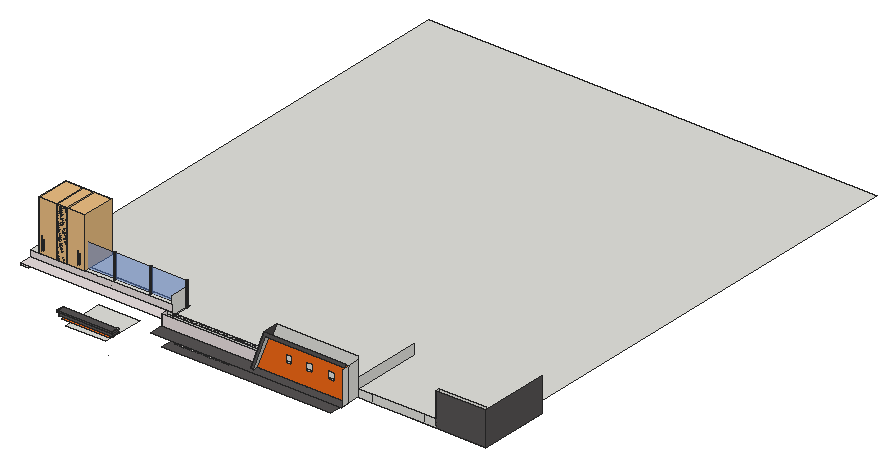
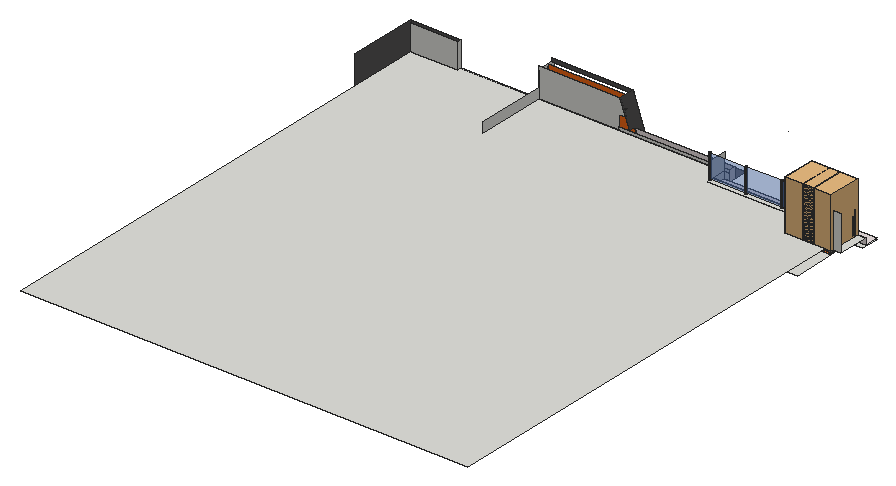
# SketchUp Ruby script. Lengths in inches.
U = 1.inch
M = Sketchup.active_model
def pt(a) = Geom::Point3d.new(a.map { |v| v * U })
def face(e, loops, mat)
  f = e.add_face(loops[0].map { |a| pt(a) })
  loops[1..].each { |l| e.add_face(l.map { |a| pt(a) }).erase! }
  f.material = f.back_material = mat if mat
  f
end
# faces: each face lists its corners as indices into pts; further lists are holes
def faces(e, pts, list, mat = nil) = list.each { |f| face(e, (f[0].is_a?(Array) ? f : [f]).map { |l| l.map { |i| pts[i] } }, mat) }
# xy, xz, yz: faces in a plane at the given z, y or x. An outline is a flat list of corners, or four numbers for a rectangle; further outlines are holes
def ring(l) = l.size == 4 ? [[l[0], l[1]], [l[2], l[1]], [l[2], l[3]], [l[0], l[3]]] : l.each_slice(2).to_a
def flat(e, list, mat, &to3) = list.each { |f| face(e, (f[0].is_a?(Array) ? f : [f]).map { |l| ring(l).map { |u, v| to3.(u, v) } }, mat) }
def xy(e, z, list, mat = nil) = flat(e, list, mat) { |x, y| [x, y, z] }
def xz(e, y, list, mat = nil) = flat(e, list, mat) { |x, z| [x, y, z] }
def yz(e, x, list, mat = nil) = flat(e, list, mat) { |y, z| [x, y, z] }
def lines(e, pts, list) = list.each { |a, b| e.add_line(pt(pts[a]), pt(pts[b])) }
# prism: a flat outline (further loops are holes) pulled along v
def prism(e, loops, v, mat = nil)
  f = face(e, loops, mat); d = Geom::Vector3d.new(v.map { |x| x * U })
  f.pushpull(f.normal.samedirection?(d) ? d.length : -d.length)
end
def box(e, o, s, mat = nil) = prism(e, [[o, [o[0] + s[0], o[1], o[2]], [o[0] + s[0], o[1] + s[1], o[2]], [o[0], o[1] + s[1], o[2]]]], [0, 0, s[2]], mat)
def at(x, y, z, deg = 0) = Geom::Transformation.translation(pt([x, y, z])) * Geom::Transformation.rotation(ORIGIN, Z_AXIS, deg.degrees)
def axes(o, x, y, z) = Geom::Transformation.new([*x, 0, *y, 0, *z, 0, *pt(o).to_a, 1])
def part(name) = M.definitions.add(name)
# library, detail: a bought-in or finely detailed component or shape, given as its bounding box
def library(name, o, s) = part(name).tap { |d| box(d.entities, o, s) }
def detail(e, o, s) = box(e.add_group.entities, o, s)
def put(e, d, t, mat = nil) = e.add_instance(d, t).tap { |i| i.material = mat if mat }
def group(e, t, mat = nil) = e.add_group.tap { |g| g.transformation = t; g.material = mat if mat }.entities
root = M.entities
M.materials.add("Generic").color = [243, 106, 23]
M.materials.add("Generic\#2").color = [87, 84, 84]
M.materials.add("Generic\#6").color = [174, 89, 41]
M.materials.add("Generic\#9").color = [233, 223, 223]
M.materials.add("[Translucent Glass Blue]").color = [100, 149, 237]
M.materials["[Translucent Glass Blue]"].alpha = 0.5
c1 = library("Plant",[-27.84,-31.84,-1.26],[68.28,70.82,154.38])
xy(root,207.139,[[115.793,121.25,154.87,162.1875]])
xy(root,211.524,[[112.407,121.25,158.881,127.4375]],"Generic")
xy(root,213.297,[[110.524,121.25,161.354,127.4375]],"Generic\#2")
xy(root,216.982,[[109.221,120,162.096,121.25]],"Generic\#2")
xy(root,217.98,[[109.165,120,162.04,127.4375]],"Generic\#2")
xy(root,231,[[220.539,107.5625,220.539,127.4375,381.97,127.4375,381.97,133.125,383.845,133.125,383.845,107.5625]],"Generic\#2")
xy(root,232.215,[[225.629,116.134,229.379,121.072],[231.317,116.134,235.067,121.072],[237.004,116.134,240.754,121.072],[242.692,116.134,246.442,121.072],[248.379,116.134,252.129,121.072],
  [254.067,116.134,257.817,121.072],[259.754,116.134,263.504,121.072],[265.442,116.134,269.192,121.072],[271.442,116.134,278.629,121.072]])
xy(root,237.6875,[[342.977,127.4375,342.977,133.364,220.539,133.364,220.539,168.255,342.977,168.255,342.977,194.75,385.914,194.75,385.914,133.125,381.97,133.125,381.97,127.4375]],"Generic\#6")
xy(root,240,[[302.78,111.75,306.093,115.8125],[302.78,115.8125,316.414,115.8125,316.414,127.4375,220.539,127.4375,220.539,120.9375,302.78,120.9375],[316.414,115.8125,394.852,127.4375],[209.664,120.9375,220.539,127.4375],[67.114,127.4375,75.375,143.9375],
  [220.539,127.4375,342.977,133.364],[381.97,127.4375,394.852,133.125],[394.852,127.4375,470.289,194.75],[[470.289,127.4375,518.6875,194.75],[472.756,133.845,475.694,136.783],[477.465,133.845,480.402,136.783],[482.59,133.845,485.527,136.783],[487.715,133.845,490.652,136.783],[492.84,133.845,495.777,136.783],[497.965,133.845,500.902,136.783],[503.09,133.845,506.027,136.783],[508.215,133.845,511.152,136.783]],[385.914,133.125,394.852,194.75]])
xy(root,240,[[209.664,107.5625,394.852,107.5625,394.852,115.8125,306.093,115.8125,306.093,111.75,302.78,111.75,302.78,120.9375,209.664,120.9375]],"Generic\#2")
xy(root,241.3125,[[80.9375,140.625,205.435,143.9375],[205.435,140.625,214.955,147.625]])
xy(root,241.3125,[[67.114,127.4375,214.955,140.625]],"Generic\#9")
xy(root,247.625,[[214.955,127.4375,470.289,127.4375,470.289,131.45,515.25,131.45,515.25,605.125,80.9375,605.125,80.9375,147.625,214.955,147.625,214.955,144.798,214.992,144.803,215.17,144.779,215.336,144.711,215.478,144.601,215.587,144.459,215.656,144.293,215.679,144.115,215.656,143.937,215.587,143.771,215.478,143.629,215.336,143.52,215.17,143.451,214.992,143.428,214.955,143.433],[67.114,140.625,214.955,140.625,214.955,143.433,214.814,143.451,214.648,143.52,214.506,143.629,214.396,143.771,214.328,143.937,214.304,144.115,214.328,144.293,214.396,144.459,180.656,144.291,180.679,144.115,180.656,143.937,180.587,143.771,180.478,143.629,180.336,143.52,180.17,143.451,179.992,143.428,179.814,143.451,179.648,143.52,179.506,143.629,179.396,143.771,179.328,143.937,179.304,144.115,179.327,144.285,145.866,144.118,145.867,144.115,145.843,143.937,145.775,143.771,145.665,143.629,145.523,143.52,145.357,143.451,145.179,143.428,145.001,143.451,144.836,143.52,144.693,143.629,144.584,143.771,144.515,143.937,144.492,144.112,111.032,143.945,111.031,143.937,110.962,143.771,110.853,143.629,110.711,143.52,110.545,143.451,110.367,143.428,110.189,143.451,110.023,143.52,109.881,143.629,109.771,143.771,109.703,143.937,109.703,143.939,76.025,143.771,75.915,143.629,75.773,143.52,75.607,143.451,75.429,143.428,75.251,143.451,75.086,143.52,74.943,143.629,74.834,143.771,74.765,143.937,74.742,144.115,74.765,144.293,74.834,144.459,74.943,144.601,75.086,144.711,75.251,144.779,75.429,144.803,75.607,144.779,75.773,144.711,75.915,144.601,76.025,144.459,76.093,144.293,76.117,144.115,76.093,143.937,76.025,143.771,109.703,143.939,109.679,144.115,109.703,144.293,109.771,144.459,109.881,144.601,110.023,144.711,110.189,144.779,110.367,144.803,110.545,144.779,110.711,144.711,110.853,144.601,110.962,144.459,111.031,144.293,111.054,144.115,111.032,143.945,144.492,144.112,144.492,144.115,144.515,144.293,144.584,144.459,144.693,144.601,144.836,144.711,145.001,144.779,145.179,144.803,145.357,144.779,145.523,144.711,145.665,144.601,145.775,144.459,145.843,144.293,145.866,144.118,179.327,144.285,179.328,144.293,179.396,144.459,179.506,144.601,179.648,144.711,179.814,144.779,179.992,144.803,180.17,144.779,180.336,144.711,180.478,144.601,180.587,144.459,180.656,144.293,180.656,144.291,214.396,144.459,214.506,144.601,214.648,144.711,214.814,144.779,214.955,144.798,214.955,147.625,80.9375,147.625,80.9375,170.6875,67.114,170.6875],[75.429,143.428,75.607,143.451,75.773,143.52,75.915,143.629,76.025,143.771,76.093,143.937,76.117,144.115,76.093,144.293,76.025,144.459,75.915,144.601,75.773,144.711,75.607,144.779,75.429,144.803,74.943,144.601,74.834,144.459,74.765,144.293,74.742,144.115,74.765,143.937,74.834,143.771,74.943,143.629,75.086,143.52,75.251,143.451],[110.367,143.428,110.545,143.451,110.711,143.52,110.853,143.629,110.962,143.771,111.031,143.937,111.032,143.945,109.703,143.939,109.703,143.937,109.771,143.771,109.881,143.629,110.023,143.52,110.189,143.451],[145.179,143.428,145.357,143.451,145.523,143.52,145.665,143.629,145.775,143.771,145.843,143.937,145.867,144.115,145.866,144.118,144.492,144.112,144.515,143.937,144.584,143.771,144.693,143.629,144.836,143.52,145.001,143.451],
  [179.992,143.428,180.17,143.451,180.336,143.52,180.478,143.629,180.587,143.771,180.656,143.937,180.679,144.115,180.656,144.291,179.327,144.285,179.304,144.115,179.328,143.937,179.396,143.771,179.506,143.629,179.648,143.52,179.814,143.451],[109.703,143.939,111.032,143.945,111.054,144.115,111.031,144.293,110.962,144.459,110.853,144.601,110.711,144.711,110.545,144.779,110.367,144.803,110.189,144.779,110.023,144.711,109.881,144.601,109.771,144.459,109.703,144.293,109.679,144.115],[144.492,144.112,145.866,144.118,145.843,144.293,145.775,144.459,145.665,144.601,145.523,144.711,145.357,144.779,145.179,144.803,145.001,144.779,144.836,144.711,144.693,144.601,144.584,144.459,144.515,144.293,144.492,144.115],[179.327,144.285,180.656,144.291,180.656,144.293,180.587,144.459,180.478,144.601,180.336,144.711,180.17,144.779,179.992,144.803,179.814,144.779,179.648,144.711,179.506,144.601,179.396,144.459,179.328,144.293],[74.943,144.601,75.429,144.803,75.251,144.779,75.086,144.711]])
xz(root,111.75,[[302.78,240,306.093,240,317.954,272.627,394.852,272.627,394.852,276.252,315.959,276.252]],"Generic\#2")
xz(root,115.8125,[[[306.093,240,394.852,240,394.852,272.627,317.954,272.627],[333.741,254.001,339.991,261.564],[353.491,254.001,359.741,261.564],[374.741,254.001,380.991,261.564]]],"Generic")
xz(root,120,[[108.098,216.919,109.221,216.982,162.096,216.982,162.782,217.02,162.709,218.331,162.022,218.292,162.04,217.98,109.165,217.98,109.147,218.292,108.024,218.229]],"Generic\#2")
xz(root,120.9375,[[209.664,240,302.78,240,306.609,250.531,209.664,250.531]],"Generic\#9")
xz(root,121.25,[[110.524,213.297,161.354,213.297,161.475,213.305,161.595,213.33,161.709,213.37,161.817,213.426,161.917,213.496,162.006,213.578,162.083,213.672,162.147,213.775,162.197,213.886,162.231,214.003,162.249,214.123,162.25,214.245,162.096,216.982,109.221,216.982,109.367,214.391,109.384,214.246,109.42,214.104,109.473,213.968,109.543,213.84,109.628,213.721,109.728,213.614,109.84,213.52,109.963,213.442,110.095,213.379,110.234,213.334,110.378,213.306]],"Generic\#2")
xz(root,127.4375,[[220.539,231,220.539,240,342.977,240,342.977,237.6875,381.97,237.6875,381.97,231],[342.977,237.6875,381.97,240],[209.664,240,209.664,241.3125,214.955,241.3125,214.955,247.625,316.414,247.625,316.414,240],[316.414,240,394.852,240,394.852,247.625,214.955,247.625,214.813,250.531,316.414,250.531],[394.852,240,407.84,247.625],
  [407.84,240,458.635,247.625],[458.635,240,470.289,247.625],[209.664,241.3125,214.955,247.625],[209.664,247.625,214.955,247.625,214.813,250.531,209.664,250.531],[214.955,247.625,316.414,247.625,316.414,250.531,214.813,250.531],
  [316.414,247.625,316.414,261.0625,310.437,261.0625,315.959,276.252,394.852,276.252,394.852,247.625]])
xz(root,127.4375,[[470.289,240,518.6875,272.4375]],"Generic\#2")
xz(root,131.45,[[470.289,247.625,515.25,272.4375]])
xz(root,133.125,[[381.97,237.6875,385.914,240]])
xz(root,133.364,[[220.539,237.6875,342.977,240]])
xz(root,140.625,[[67.114,241.3125,214.955,247.625]],"Generic\#9")
xz(root,143.9375,[[80.9375,240,205.435,241.3125]])
xz(root,147.625,[[145.165,243.8125,180.06,247.625]])
xz(root,168.255,[[220.539,237.6875,342.977,240]])
xz(root,170.6875,[[67.114,247.625,77.5625,281.899]])
yz(root,74.943,[[144.601,247.828,171.546,270.251]],"[Translucent Glass Blue]")
yz(root,209.664,[[120.9375,240,127.4375,250.531]],"Generic\#9")
yz(root,214.955,[[127.4375,241.3125,140.625,247.625]])
yz(root,342.977,[[127.4375,237.6875,133.364,240]])
yz(root,381.97,[[127.4375,231,133.125,237.6875],[127.4375,237.6875,133.125,240]])
yz(root,385.914,[[133.125,237.6875,194.75,240]])
yz(root,394.852,[[108.375,240,115.8125,272.627],[115.8125,240,127.4375,272.627],[127.4375,240,194.75,256.5625]])
yz(root,470.289,[[127.4375,247.625,131.45,272.4375]])
yz(root,518.6875,[[127.4375,240,194.75,272.4375]],"Generic\#2")
p = [[110.095,127.4375,213.379],[110.234,127.4375,213.334],[110.234,121.25,213.334],[110.095,121.25,213.379],[110.378,127.4375,213.306],[110.378,121.25,213.306],
  [110.524,127.4375,213.297],[110.524,121.25,213.297],[161.354,127.4375,213.297],[161.475,127.4375,213.305],[161.475,121.25,213.305],[161.354,121.25,213.297],
  [161.595,127.4375,213.33],[161.595,121.25,213.33],[161.709,127.4375,213.37],[161.709,121.25,213.37],[109.84,127.4375,213.52],[109.963,127.4375,213.442],
  [109.963,121.25,213.442],[109.84,121.25,213.52],[161.817,127.4375,213.426],[161.817,121.25,213.426],[161.917,127.4375,213.496],[161.917,121.25,213.496],
  [109.728,127.4375,213.614],[109.728,121.25,213.614],[162.006,127.4375,213.578],[162.006,121.25,213.578],[109.628,127.4375,213.721],[109.628,121.25,213.721],
  [162.083,127.4375,213.672],[162.083,121.25,213.672],[109.543,127.4375,213.84],[109.543,121.25,213.84],[162.147,127.4375,213.775],[162.147,121.25,213.775],
  [109.473,127.4375,213.968],[109.473,121.25,213.968],[162.197,127.4375,213.886],[162.197,121.25,213.886],[162.231,127.4375,214.003],[162.231,121.25,214.003],
  [109.42,127.4375,214.104],[109.42,121.25,214.104],[162.249,127.4375,214.123],[162.249,121.25,214.123],[109.384,127.4375,214.246],[109.384,121.25,214.246],
  [162.25,127.4375,214.245],[162.25,121.25,214.245],[109.367,127.4375,214.391],[109.367,121.25,214.391],[162.096,127.4375,216.982],[162.096,121.25,216.982],
  [109.221,127.4375,216.982],[109.221,121.25,216.982],[108.024,127.4375,218.229],[108.098,127.4375,216.919],[108.098,121.25,216.919],[108.098,120,216.919],
  [108.024,120,218.229],[109.221,120,216.982],[162.096,120,216.982],[162.782,121.25,217.02],[162.782,120,217.02],[162.782,127.4375,217.02],
  [162.709,127.4375,218.331],[162.709,120,218.331],[109.165,120,217.98],[109.165,127.4375,217.98],[109.147,127.4375,218.292],[109.147,120,218.292],
  [162.04,127.4375,217.98],[162.04,120,217.98],[162.022,120,218.292],[162.022,127.4375,218.292],[302.78,115.8125,240],[302.78,111.75,240],
  [315.959,111.75,276.252],[315.959,115.8125,276.252],[315.959,127.4375,276.252],[310.437,127.4375,261.0625],[306.609,127.4375,250.531],[306.609,124.118,250.531],
  [306.609,120.9375,250.531],[302.78,120.9375,240],[312.685,123.307,267.247],[312.403,123.237,266.469],[311.912,123.115,265.119],[311.912,126.052,265.119],
  [312.403,126.175,266.469],[312.685,126.245,267.247],[306.093,115.8125,240],[317.954,115.8125,272.627],[317.954,111.75,272.627],[306.093,111.75,240],
  [214.955,143.103,247.625],[214.101,143.103,265.119],[214.101,127.4375,265.119],[214.813,127.4375,250.531],[214.955,127.4375,247.625],[214.955,140.625,247.625],
  [75.251,143.451,247.625],[75.429,143.428,247.625],[75.429,143.428,271.3125],[75.251,143.451,271.3125],[75.607,143.451,247.625],[75.607,143.451,271.3125],
  [110.189,143.451,247.625],[110.367,143.428,247.625],[110.367,143.428,271.3125],[110.189,143.451,271.3125],[110.545,143.451,247.625],[110.545,143.451,271.3125],
  [145.001,143.451,247.625],[145.179,143.428,247.625],[145.179,143.428,271.3125],[145.001,143.451,271.3125],[145.357,143.451,247.625],[145.357,143.451,271.3125],
  [179.814,143.451,247.625],[179.992,143.428,247.625],[179.992,143.428,271.3125],[179.814,143.451,271.3125],[180.17,143.451,247.625],[180.17,143.451,271.3125],
  [214.814,143.451,247.625],[214.955,143.433,247.625],[214.955,143.433,266.469],[214.955,143.433,271.3125],[214.814,143.451,271.3125],[214.992,143.428,247.625],
  [214.992,143.428,271.3125],[215.17,143.451,247.625],[215.17,143.451,271.3125],[74.943,143.629,247.625],[75.086,143.52,247.625],[75.086,143.52,271.3125],
  [74.943,143.629,271.3125],[75.773,143.52,247.625],[75.773,143.52,271.3125],[75.915,143.629,247.625],[75.915,143.629,271.3125],[109.881,143.629,247.625],
  [110.023,143.52,247.625],[110.023,143.52,271.3125],[109.881,143.629,271.3125],[110.711,143.52,247.625],[110.711,143.52,271.3125],[110.853,143.629,247.625],
  [110.853,143.629,271.3125],[144.693,143.629,247.625],[144.836,143.52,247.625],[144.836,143.52,271.3125],[144.693,143.629,271.3125],[145.523,143.52,247.625],
  [145.523,143.52,271.3125],[145.665,143.629,247.625],[145.665,143.629,271.3125],[179.506,143.629,247.625],[179.648,143.52,247.625],[179.648,143.52,271.3125],
  [179.506,143.629,271.3125],[180.336,143.52,247.625],[180.336,143.52,271.3125],[180.478,143.629,247.625],[180.478,143.629,271.3125],[214.506,143.629,247.625],
  [214.648,143.52,247.625],[214.648,143.52,271.3125],[214.506,143.629,271.3125],[215.336,143.52,247.625],[215.336,143.52,271.3125],[215.478,143.629,247.625],
  [215.478,143.629,271.3125],[74.834,143.771,247.625],[74.834,143.771,271.3125],[76.025,143.771,247.625],[76.025,143.771,271.3125],[109.771,143.771,247.625],
  [109.771,143.771,271.3125],[110.962,143.771,247.625],[110.962,143.771,271.3125],[144.584,143.771,247.625],[144.584,143.771,271.3125],[145.775,143.771,247.625],
  [145.775,143.771,271.3125],[179.396,143.771,247.625],[179.396,143.771,271.3125],[180.587,143.771,247.625],[180.587,143.771,271.3125],[214.396,143.771,247.625],
  [214.396,143.771,271.3125],[215.587,143.771,247.625],[215.587,143.771,271.3125],[74.765,143.937,247.625],[74.765,143.937,271.3125],[76.093,143.937,247.625],
  [76.093,143.937,271.3125],[109.703,143.939,271.3125],[111.032,143.945,271.3125],[144.492,144.112,271.3125],[145.866,144.118,271.3125],[179.327,144.285,271.3125],
  [180.656,144.291,271.3125],[214.396,144.459,271.3125],[214.396,144.459,247.625],[180.656,144.291,247.625],[179.327,144.285,247.625],[145.866,144.118,247.625],
  [144.492,144.112,247.625],[111.032,143.945,247.625],[109.703,143.939,247.625],[109.703,143.937,247.625],[109.703,143.937,271.3125],[111.031,143.937,247.625],
  [111.031,143.937,271.3125],[144.515,143.937,247.625],[144.515,143.937,271.3125],[145.843,143.937,247.625],[145.843,143.937,271.3125],[179.328,143.937,247.625],
  [179.328,143.937,271.3125],[180.656,143.937,247.625],[180.656,143.937,271.3125],[214.328,143.937,247.625],[214.328,143.937,271.3125],[215.656,143.937,247.625],
  [215.656,143.937,271.3125],[74.742,144.115,247.625],[74.742,144.115,271.3125],[76.117,144.115,247.625],[76.117,144.115,271.3125],[109.679,144.115,271.3125],
  [109.679,144.115,247.625],[111.054,144.115,247.625],[111.054,144.115,271.3125],[144.492,144.115,271.3125],[144.492,144.115,247.625],[145.867,144.115,247.625],
  [145.867,144.115,271.3125],[179.304,144.115,247.625],[179.304,144.115,271.3125],[180.679,144.115,247.625],[180.679,144.115,271.3125],[214.304,144.115,247.625],
  [214.304,144.115,271.3125],[215.679,144.115,247.625],[215.679,144.115,271.3125],[74.765,144.293,247.625],[74.765,144.293,271.3125],[76.093,144.293,247.625],
  [76.093,144.293,271.3125],[109.703,144.293,247.625],[109.703,144.293,271.3125],[111.031,144.293,247.625],[111.031,144.293,271.3125],[144.515,144.293,247.625],
  [144.515,144.293,271.3125],[145.843,144.293,247.625],[145.843,144.293,271.3125],[179.328,144.293,271.3125],[179.328,144.293,247.625],[180.656,144.293,247.625],
  [180.656,144.293,271.3125],[214.328,144.293,247.625],[214.328,144.293,271.3125],[215.656,144.293,247.625],[215.656,144.293,271.3125],[74.834,144.459,247.625],
  [74.834,144.459,271.3125],[76.025,144.459,247.625],[76.025,144.459,271.3125],[109.771,144.459,247.625],[109.771,144.459,271.3125],[110.962,144.459,247.625],
  [110.962,144.459,271.3125],[144.584,144.459,247.625],[144.584,144.459,271.3125],[145.775,144.459,247.625],[145.775,144.459,271.3125],[179.396,144.459,247.625],
  [179.396,144.459,271.3125],[180.587,144.459,247.625],[180.587,144.459,271.3125],[215.587,144.459,247.625],[215.587,144.459,271.3125],[74.943,144.601,247.625],
  [74.943,144.601,271.3125],[74.943,144.601,270.251],[74.943,144.601,247.828],[75.915,144.601,247.625],[75.915,144.601,271.3125],[109.881,144.601,247.625],
  [109.881,144.601,271.3125],[110.853,144.601,247.625],[110.853,144.601,271.3125],[144.693,144.601,247.625],[144.693,144.601,271.3125],[145.665,144.601,247.625],
  [145.665,144.601,271.3125],[179.506,144.601,247.625],[179.506,144.601,271.3125],[180.478,144.601,247.625],[180.478,144.601,271.3125],[214.506,144.601,247.625],
  [214.506,144.601,271.3125],[215.478,144.601,247.625],[215.478,144.601,271.3125],[75.086,144.711,247.625],[75.086,144.711,271.3125],[75.429,144.803,247.625],
  [75.429,144.803,270.251],[75.773,144.711,247.625],[75.773,144.711,271.3125],[110.023,144.711,247.625],[110.023,144.711,271.3125],[110.711,144.711,247.625],
  [110.711,144.711,271.3125],[144.836,144.711,247.625],[144.836,144.711,271.3125],[145.523,144.711,247.625],[145.523,144.711,271.3125],[179.648,144.711,247.625],
  [179.648,144.711,271.3125],[180.336,144.711,247.625],[180.336,144.711,271.3125],[214.648,144.711,247.625],[214.648,144.711,271.3125],[215.336,144.711,247.625],
  [215.336,144.711,271.3125],[75.251,144.779,247.625],[75.251,144.779,271.3125],[75.607,144.779,247.625],[75.607,144.779,271.3125],[110.189,144.779,247.625],
  [110.189,144.779,271.3125],[110.545,144.779,247.625],[110.545,144.779,271.3125],[145.001,144.779,247.625],[145.001,144.779,271.3125],[145.357,144.779,247.625],
  [145.357,144.779,271.3125],[179.814,144.779,247.625],[179.814,144.779,271.3125],[180.17,144.779,247.625],[180.17,144.779,271.3125],[214.814,144.779,247.625],
  [214.814,144.779,271.3125],[215.17,144.779,247.625],[215.17,144.779,271.3125],[75.429,144.803,271.3125],[110.367,144.803,247.625],[110.367,144.803,271.3125],
  [145.179,144.803,247.625],[145.179,144.803,271.3125],[179.992,144.803,247.625],[179.992,144.803,271.3125],[214.955,144.798,247.625],[214.955,144.798,271.3125],
  [214.992,144.803,247.625],[214.992,144.803,271.3125],[470.289,131.45,247.625],[470.289,131.75,247.625],[220.539,133.364,240],[220.539,168.255,240],
  [205.435,143.9375,240],[205.435,127.4375,240],[214.955,143.9375,247.625],[214.955,143.9375,266.469],[180.06,143.9375,247.625],[180.06,143.9375,266.469],
  [145.165,143.9375,247.625],[145.165,143.9375,266.469],[110.27,143.9375,247.625],[110.27,143.9375,266.469],[75.375,143.9375,247.625],[75.375,143.9375,266.469],
  [73.625,143.9375,241.3125],[80.9375,143.9375,241.3125],[75.375,147.625,241.3125],[205.435,147.625,241.3125],[214.955,147.625,247.625],[214.955,147.625,241.3125],
  [145.165,140.625,243.8125],[145.165,147.625,243.8125],[214.955,48.734,247.625],[214.955,49.354,247.625]]
faces(root,p,[[0,1,2,3],[1,4,5,2],[4,6,7,5],[8,9,10,11],[9,12,13,10],[12,14,15,13],[16,17,18,19],[17,0,3,18],
  [14,20,21,15],[20,22,23,21],[24,16,19,25],[22,26,27,23],[28,24,25,29],[26,30,31,27],[32,28,29,33],[30,34,35,31],
  [36,32,33,37],[34,38,39,35],[38,40,41,39],[42,36,37,43],[40,44,45,41],[46,42,43,47],[44,48,49,45],[50,46,47,51],
  [48,52,53,49],[54,50,51,55],[56,57,58,59,60],[55,61,59,58],[54,55,58,57],[62,53,63,64],[65,66,67,64,63],[53,52,65,63],
  [[76,77,78,79,80,81,82,83,84,85],[86,87,88,89,90,91]]],"Generic\#2")
faces(root,p,[[68,69,70,71],[72,73,74,75],[71,70,56,60],[75,74,67,66],[92,93,94,95],[96,97,98,99,100,101],[102,103,104,105],[103,106,107,104],
  [108,109,110,111],[109,112,113,110],[114,115,116,117],[115,118,119,116],[120,121,122,123],[121,124,125,122],[126,127,128,129,130],[127,131,132,129,128],
  [131,133,134,132],[135,136,137,138],[136,102,105,137],[106,139,140,107],[139,141,142,140],[143,144,145,146],[144,108,111,145],[112,147,148,113],
  [147,149,150,148],[151,152,153,154],[152,114,117,153],[118,155,156,119],[155,157,158,156],[159,160,161,162],[160,120,123,161],[124,163,164,125],
  [163,165,166,164],[167,168,169,170],[168,126,130,169],[133,171,172,134],[171,173,174,172],[175,135,138,176],[141,177,178,142],[179,143,146,180],
  [149,181,182,150],[183,151,154,184],[157,185,186,158],[187,159,162,188],[165,189,190,166],[191,167,170,192],[173,193,194,174],[195,175,176,196],
  [177,197,198,178],[213,179,180,214],[181,215,216,182],[217,183,184,218],[185,219,220,186],[221,187,188,222],[189,223,224,190],[225,191,192,226],
  [193,227,228,194],[229,195,196,230],[197,231,232,198],[212,213,214,199,233,234],[211,235,236,200,216,215],[210,217,218,201,237,238],[219,239,240,220],[241,221,222,242],
  [223,243,244,224],[245,225,226,246],[227,247,248,228],[249,229,230,250],[231,251,252,232],[253,234,233,254],[235,255,256,236],[257,238,237,258],
  [209,259,260,202,240,239],[208,241,242,203,261,262],[207,263,264,204,244,243],[265,245,246,266],[247,267,268,248],[269,249,250,270],[251,271,272,252],[273,253,254,274],
  [255,275,276,256],[277,257,258,278],[259,279,280,260],[281,262,261,282],[263,283,284,264],[206,265,266,205],[267,285,286,268],[287,269,270,288,289,290],
  [271,291,292,272],[293,273,274,294],[275,295,296,276],[297,277,278,298],[279,299,300,280],[301,281,282,302],[283,303,304,284],[305,206,205,306],
  [285,307,308,286],[309,287,290,289,288,310],[311,287,290,289,312],[291,313,314,292],[315,293,294,316],[295,317,318,296],[319,297,298,320],[299,321,322,300],
  [323,301,302,324],[303,325,326,304],[327,305,306,328],[307,329,330,308],[331,309,310,332],[313,333,334,314],[335,315,316,336],[317,337,338,318],
  [339,319,320,340],[321,341,342,322],[343,323,324,344],[325,345,346,326],[347,327,328,348],[329,349,350,330],[311,331,332,351,312],[333,311,312,351,334],
  [352,335,336,353],[337,352,353,338],[354,339,340,355],[341,354,355,342],[356,343,344,357],[345,356,357,346],[358,347,348,359],[349,360,361,350],
  [360,358,359,361]])
faces(root,p,[[177,178,199,200,201,202,203,204,205,206,207,208,209,210,211,212]],"[Translucent Glass Blue]")
lines(root,p,[[362,363],[364,365],[366,367],[368,369],[370,371],[372,373],[374,375],[376,377],[378,379],[380,381],[382,383],[384,385],
  [386,387]])
put(root,c1,axes([86.15,154.72,247.83],[0.40581,0,0],[0,0.45951,0],[0,0,0.31484]))
put(root,c1,axes([103.34,154.72,247.83],[0.40581,0,0],[0,0.45951,0],[0,0,0.31484]))
